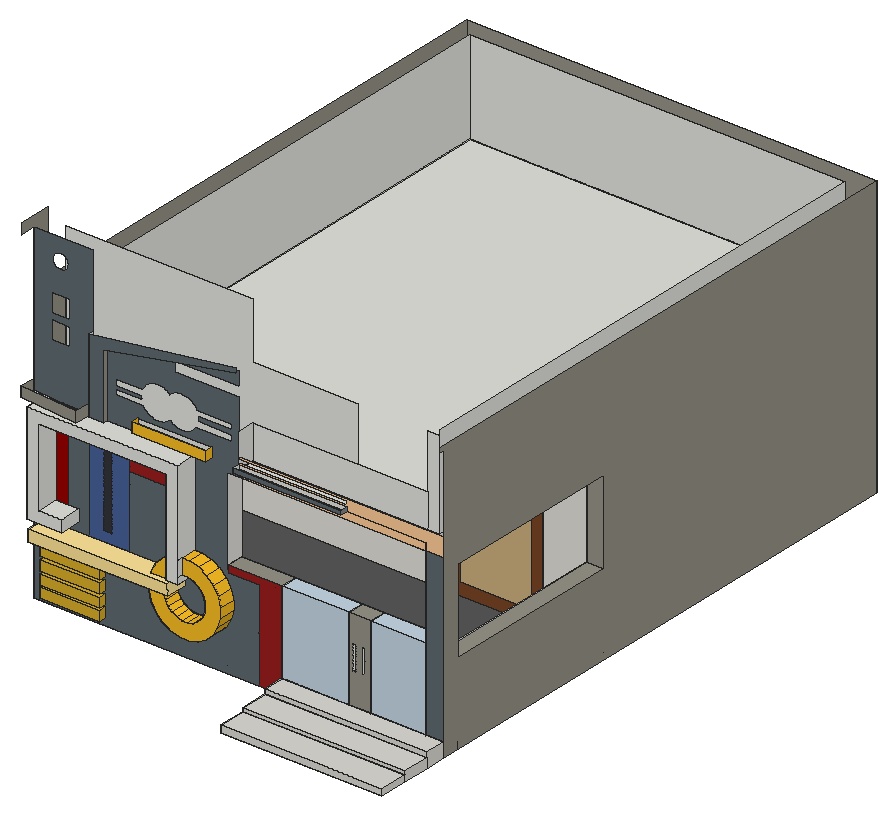
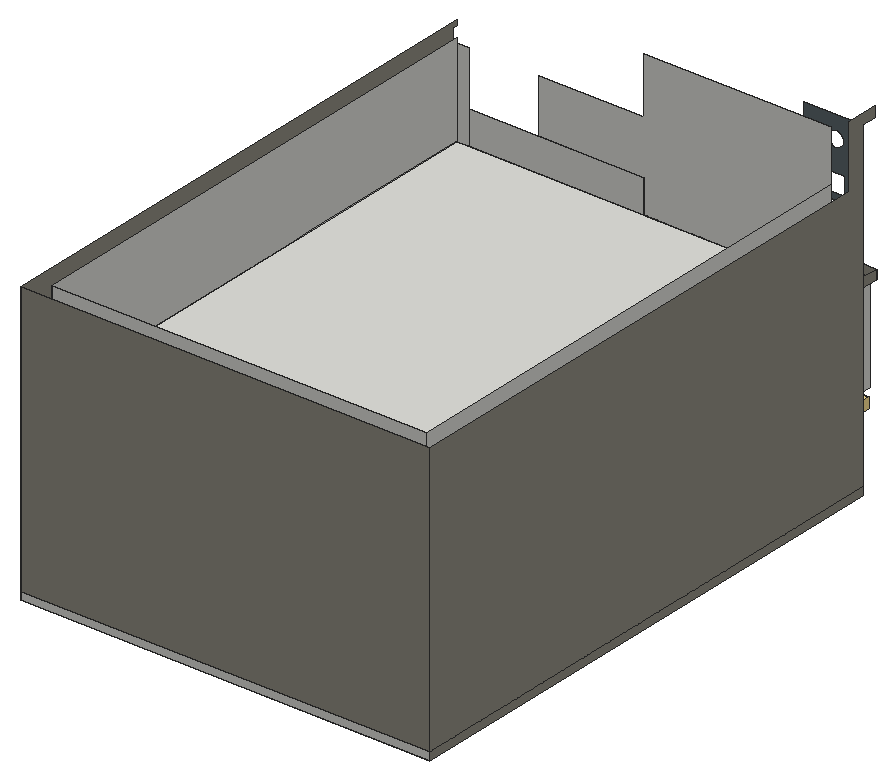
# SketchUp Ruby script. Lengths in inches.
U = 1.inch
M = Sketchup.active_model
def pt(a) = Geom::Point3d.new(a.map { |v| v * U })
def face(e, loops, mat)
  f = e.add_face(loops[0].map { |a| pt(a) })
  loops[1..].each { |l| e.add_face(l.map { |a| pt(a) }).erase! }
  f.material = f.back_material = mat if mat
  f
end
# faces: each face lists its corners as indices into pts; further lists are holes
def faces(e, pts, list, mat = nil) = list.each { |f| face(e, (f[0].is_a?(Array) ? f : [f]).map { |l| l.map { |i| pts[i] } }, mat) }
# xy, xz, yz: faces in a plane at the given z, y or x. An outline is a flat list of corners, or four numbers for a rectangle; further outlines are holes
def ring(l) = l.size == 4 ? [[l[0], l[1]], [l[2], l[1]], [l[2], l[3]], [l[0], l[3]]] : l.each_slice(2).to_a
def flat(e, list, mat, &to3) = list.each { |f| face(e, (f[0].is_a?(Array) ? f : [f]).map { |l| ring(l).map { |u, v| to3.(u, v) } }, mat) }
def xy(e, z, list, mat = nil) = flat(e, list, mat) { |x, y| [x, y, z] }
def xz(e, y, list, mat = nil) = flat(e, list, mat) { |x, z| [x, y, z] }
def yz(e, x, list, mat = nil) = flat(e, list, mat) { |y, z| [x, y, z] }
def lines(e, pts, list) = list.each { |a, b| e.add_line(pt(pts[a]), pt(pts[b])) }
# prism: a flat outline (further loops are holes) pulled along v
def prism(e, loops, v, mat = nil)
  f = face(e, loops, mat); d = Geom::Vector3d.new(v.map { |x| x * U })
  f.pushpull(f.normal.samedirection?(d) ? d.length : -d.length)
end
def box(e, o, s, mat = nil) = prism(e, [[o, [o[0] + s[0], o[1], o[2]], [o[0] + s[0], o[1] + s[1], o[2]], [o[0], o[1] + s[1], o[2]]]], [0, 0, s[2]], mat)
def at(x, y, z, deg = 0) = Geom::Transformation.translation(pt([x, y, z])) * Geom::Transformation.rotation(ORIGIN, Z_AXIS, deg.degrees)
def axes(o, x, y, z) = Geom::Transformation.new([*x, 0, *y, 0, *z, 0, *pt(o).to_a, 1])
def part(name) = M.definitions.add(name)
# library, detail: a bought-in or finely detailed component or shape, given as its bounding box
def library(name, o, s) = part(name).tap { |d| box(d.entities, o, s) }
def detail(e, o, s) = box(e.add_group.entities, o, s)
def put(e, d, t, mat = nil) = e.add_instance(d, t).tap { |i| i.material = mat if mat }
def group(e, t, mat = nil) = e.add_group.tap { |g| g.transformation = t; g.material = mat if mat }.entities
root = M.entities
M.materials.add("[0045_Goldenrod]").color = [249, 189, 36]
M.materials.add("[Blacktop Old 01]").color = [132, 136, 139]
M.materials.add("[Carpet Plush Charcoal]").color = [87, 87, 87]
M.materials.add("[Color A04]").color = [155, 30, 30]
M.materials.add("[Color A07]").color = [153, 0, 0]
M.materials.add("[Color C02]").color = [255, 204, 153]
M.materials.add("[Color D02]").color = [255, 229, 153]
M.materials.add("[Color D04]").color = [216, 173, 42]
M.materials.add("[Formica Blue]").color = [71, 97, 152]
M.materials.add("[Formica Graystone]").color = [149, 146, 135]
M.materials.add("[Formica Laminate Dark]").color = [50, 53, 60]
M.materials.add("[Formica Speckled Grey]").color = [94, 105, 111]
M.materials.add("[Marble Carrara Gold Floor Tile]").color = [225, 223, 217]
M.materials.add("[Terrazzo Light Blue]").color = [196, 214, 227]
M.materials.add("[Terrazzo Tile Light]").color = [219, 217, 210]
M.materials.add("[Window Covering 02]").color = [199, 178, 115]
M.materials.add("[Wood Bamboo]").color = [177, 105, 43]
M.materials.add("[Wood Floor Light]").color = [204, 176, 127]
M.materials.add("[Wood Veneer 01]").color = [120, 70, 37]
M.materials.add("[Wood Veneer 02]").color = [190, 128, 91]
xy(root,0,[[307.14,0,506.36,34.29],[307.14,34.29,506.36,68.57],[307.14,68.57,506.36,94.74],[1.43,94.74,506.36,761.28]])
xy(root,7.65,[[14.67,86.37,88.61,94.74]])
xy(root,8.0625,[[307.14,0,506.36,34.29]],"[Terrazzo Tile Light]")
xy(root,9,[[307.14,94.74,389.07,116.19],[389.07,94.74,416.47,116.19],[416.47,94.74,484.91,116.19],[22.875,341.3,314.74,362.64],[314.74,341.3,431.36,362.64],
  [431.36,341.3,484.91,362.64],[22.875,362.64,484.91,739.83]])
xy(root,9,[[22.875,116.19,484.91,341.3]],"[Carpet Plush Charcoal]")
xy(root,12.25,[[307.14,34.29,506.36,68.57]],"[Terrazzo Tile Light]")
xy(root,18.125,[[307.14,68.57,506.36,94.74]],"[Terrazzo Tile Light]")
xy(root,19.77,[[14.67,86.37,88.61,94.74]],"[Color D04]")
xy(root,22.33,[[14.67,86.37,88.61,94.74]])
xy(root,34.46,[[14.67,86.37,88.61,94.74]],"[Color D04]")
xy(root,38.08,[[14.67,86.37,88.61,94.74]])
xy(root,50.21,[[14.67,86.37,88.61,94.74]],"[Color D04]")
xy(root,53.83,[[14.67,86.37,88.61,94.74]])
xy(root,65.96,[[14.67,86.37,88.61,94.74]],"[Color D04]")
xy(root,78.48,[[15.3,67.74,158.3125,94.74],[158.3125,67.74,177.44,75.3],[177.44,67.74,187.4,94.74]])
xy(root,89.58,[[129.59,341.3,239.96,362.64]])
xy(root,92.04,[[15.3,67.74,187.09,67.74,187.09,94.74,181.82,94.74,181.82,75.3,160.61,75.3,160.61,94.74,15.3,94.74]],"[Color D02]")
xy(root,96,[[185.25,67.74,199.68,94.74]])
xy(root,101,[[484.91,116.19,506.36,341.3]],"[Formica Graystone]")
xy(root,103.04,[[14.18,67.74,56.82,94.74]])
xy(root,117.47,[[28.61,67.74,56.82,94.74]])
xy(root,119.8125,[[240.02,94.74,307.14,116.19],[389.07,94.74,416.47,116.19]],"[Formica Graystone]")
xy(root,119.8125,[[307.14,94.74,389.07,116.19],[416.47,94.74,484.91,116.19]],"[Terrazzo Light Blue]")
xy(root,191.83,[[129.59,341.3,239.96,362.64]])
xy(root,197.7,[[314.74,341.3,431.36,362.64]])
xy(root,205.0625,[[484.91,116.19,506.36,341.3]],"[Formica Graystone]")
xy(root,212.8,[[28.61,67.74,44.09,94.74],[44.09,67.74,69.22,94.74],[69.22,67.74,118.93,94.74],[118.93,67.74,185.25,94.74]])
xy(root,221.375,[[253.89,94.74,253.89,116.19,22.875,116.19,22.875,341.3,484.91,341.3,484.91,94.74],[240.02,94.74,253.89,116.19],[22.875,341.3,484.91,362.64],[22.875,362.64,484.91,739.83]])
xy(root,227.23,[[14.18,67.74,199.68,67.74,199.68,94.74,91.53,94.74,91.53,89.43,73.65,89.43,14.18,93.8],[73.65,89.43,73.65,94.74,14.18,94.74,14.18,93.8],[73.65,89.43,91.53,94.74]])
xy(root,230.375,[[253.89,94.74,470.23,116.19],[470.23,94.74,484.91,116.19],[22.875,116.19,484.91,739.83]])
xy(root,230.375,[[253.89,85.74,386.77,94.74]],"[Blacktop Old 01]")
xy(root,230.54,[[129.08,85.18,220.21,94.74]],"[0045_Goldenrod]")
xz(root,0,[[307.14,0,506.36,8.0625]],"[Terrazzo Tile Light]")
xz(root,34.29,[[307.14,0,506.36,8.0625]])
xz(root,34.29,[[307.14,8.0625,506.36,12.25]],"[Terrazzo Tile Light]")
xz(root,67.74,[[185.25,96,199.68,96,199.68,227.23,14.18,227.23,14.18,103.04,56.82,103.04,56.82,117.47,28.61,117.47,28.61,212.8,185.25,212.8]])
xz(root,67.74,[[15.3,78.48,187.4,78.48,187.09,92.04,15.3,92.04]],"[Color D02]")
xz(root,68.57,[[307.14,0,506.36,12.25]])
xz(root,68.57,[[307.14,12.25,506.36,18.125]],"[Terrazzo Tile Light]")
xz(root,75.3,[[208.09,33.22,219.43,36.12,229.62,41.86,237.98,50.04,243.94,60.1,247.1,71.37,247.22,83.07,244.32,94.4,238.58,104.6,230.4,112.96,220.34,118.92,209.07,122.07,199.68,122.17,199.68,103.04,206.34,102.97,212.76,101.17,218.49,97.78,223.15,93.02,226.41,87.21,228.07,80.76,227.99,74.1,226.2,67.68,222.81,61.95,218.04,57.29,212.24,54.03,205.79,52.375,199.125,52.45,192.71,54.24,186.98,57.64,182.32,62.4,179.05,68.2,177.4,74.66,177.44,78.48,158.3125,78.48,158.24,72.35,161.15,61.02,166.88,50.82,175.0625,42.46,185.13,36.5,196.4,33.35],[160.61,92.04,181.82,92.04,182.66,93.46,185.25,96,185.25,118.85,175.85,113.56,167.48,105.38,166.1,103.04,161.52,95.3125]],"[0045_Goldenrod]")
xz(root,85.18,[[129.08,230.54,220.21,243.23]],"[0045_Goldenrod]")
xz(root,85.74,[[253.89,230.375,386.77,235.375]],"[Formica Speckled Grey]")
xz(root,86.37,[[14.67,7.65,88.61,19.77],[14.67,22.33,88.61,34.46],[14.67,38.08,88.61,50.21],[14.67,53.83,88.61,65.96]],"[Color D04]")
xz(root,89.43,[[73.65,227.23,91.53,227.23,91.53,307.22,253.89,338.91,253.89,345.125,73.65,318.75]],"[Formica Speckled Grey]")
xz(root,94.74,[[[208.09,33.22,219.43,36.12,229.62,41.86,237.98,50.04,243.94,60.1,247.1,71.37,247.22,83.07,244.32,94.4,238.58,104.6,230.4,112.96,220.34,118.92,209.07,122.07,199.68,122.17,199.68,227.23,14.18,227.23,14.18,103.04,56.82,103.04,56.82,117.47,28.61,117.47,28.61,212.8,185.25,212.8,185.25,118.85,175.85,113.56,167.48,105.38,166.1,103.04,161.52,95.3125,160.61,92.04,15.3,92.04,15.3,78.48,158.3125,78.48,158.24,72.35,161.15,61.02,166.88,50.82,175.0625,42.46,185.13,36.5,196.4,33.35],[205.79,52.375,199.125,52.45,192.71,54.24,186.98,57.64,182.32,62.4,179.05,68.2,177.4,74.66,177.44,78.48,187.4,78.48,187.09,92.04,181.82,92.04,182.66,93.46,185.25,96,199.68,96,199.68,103.04,206.34,102.97,212.76,101.17,218.49,97.78,223.15,93.02,226.41,87.21,228.07,80.76,227.99,74.1,226.2,67.68,222.81,61.95,218.04,57.29,212.24,54.03]],[394.31,57.13,398.19,87.45],[405.38,57.13,409.25,87.45],[253.89,230.375,386.77,235.375]])
xz(root,94.74,[[278.8125,0,307.14,0,307.14,119.8125,240.02,119.8125,240.02,111.5,278.8125,111.5],[118.93,179.99,185.25,212.8]],"[Color A04]")
xz(root,94.74,[[28.61,117.47,44.09,212.8]],"[Color A07]")
xz(root,94.74,[[253.89,221.375,484.91,230.375],[484.91,221.375,506.36,221.375,506.36,243.88,253.89,243.88,253.89,242.13,386.77,242.13,386.77,237.13,253.89,237.13,253.89,235.375,386.77,235.375,386.77,230.375,484.91,230.375]],"[Color C02]")
xz(root,94.74,[[[69.22,92.04,118.93,212.8],[86.91,104.33,97.34,197.21]]],"[Formica Blue]")
xz(root,94.74,[[389.07,9,416.47,18.125],[[389.07,18.125,416.47,119.8125],[394.31,57.13,398.19,87.45],[405.38,57.13,409.25,87.45]]],"[Formica Graystone]")
xz(root,94.74,[[86.91,104.33,97.34,197.21]],"[Formica Laminate Dark]")
xz(root,94.74,[[[1.43,0,278.8125,0,278.8125,111.5,240.02,111.5,240.02,221.375,253.89,221.375,253.89,310.29,175.33,310.29,175.33,322.92,253.89,322.92,253.89,338.91,91.53,307.22,91.53,227.23,199.68,227.23,199.68,122.17,209.07,122.07,220.34,118.92,230.4,112.96,238.58,104.6,244.32,94.4,247.22,83.07,247.1,71.37,243.94,60.1,237.98,50.04,229.62,41.86,219.43,36.12,208.09,33.22,196.4,33.35,185.13,36.5,175.0625,42.46,166.88,50.82,161.15,61.02,158.24,72.35,158.3125,78.48,15.3,78.48,15.3,92.04,69.22,92.04,69.22,212.8,44.09,212.8,44.09,117.47,56.82,117.47,56.82,103.04,14.18,103.04,14.18,227.23,73.65,227.23,73.65,408.81,1.43,408.81],[153.66,248.1,151.5,248.25,149.38,248.64,147.3,249.24,145.31,250.05,143.4,251.07,141.62,252.28,139.97,253.68,138.47,255.23,137.15,256.9375,136.0625,258.6875,102.1,258.6875,102.1,265.74,133.7,265.74,133.53,266.98,133.46,269.14,133.48,269.39,101.95,269.39,101.95,276.95,135.19,276.95,135.41,277.49,136.43,279.39,137.64,281.18,139.04,282.83,140.59,284.32,142.3,285.65,144.13,286.79,146.08,287.73,148.11,288.46,150.2,288.98,152.34,289.27,154.5,289.34,156.65,289.18,158.78,288.8,160.85,288.2,162.85,287.38,164.75,286.36,166.54,285.15,168.19,283.76,168.82,283.1,170.09,284.32,171.8,285.65,173.63,286.79,175.58,287.73,177.61,288.46,179.7,288.98,181.84,289.27,184,289.34,186.15,289.18,188.28,288.8,190.35,288.2,192.35,287.38,194.25,286.36,196.04,285.15,197.69,283.76,199.19,282.2,200.51,280.5,201.65,278.66,202,277.9375,245.58,277.9375,245.58,270.5625,204.12,270.5625,204.13,270.45,204.2,268.3,204.08,266.6,204.04,266.14,203.97,265.74,245.58,265.74,245.58,257.2,200.65,257.2,200.01,256.26,198.62,254.61,197.0625,253.11,195.36,251.79,193.52,250.65,191.58,249.71,189.55,248.98,187.45,248.46,185.3125,248.17,183.16,248.1,181,248.25,178.88,248.64,176.8,249.24,174.81,250.05,172.9,251.07,171.12,252.28,169.47,253.68,168.84,254.33,167.5625,253.11,165.86,251.79,164.02,250.65,162.08,249.71,160.05,248.98,157.95,248.46,155.8125,248.17],[129.08,230.54,220.21,243.23],[14.67,53.83,88.61,65.96],[14.67,38.08,88.61,50.21],[14.67,22.33,88.61,34.46],[14.67,7.65,88.61,19.77],[23.1,292.05,45.78,314.74],[23.1,322.3,45.78,344.99],[34.11,372.72,31.62,373.05,29.3,374.01,27.3,375.54,25.78,377.53,24.8125,379.85,24.49,382.34,24.8125,384.83,25.78,387.15,27.3,389.15,29.3,390.68,31.62,391.64,34.11,391.97,36.6,391.64,38.92,390.68,40.92,389.15,42.45,387.15,43.41,384.83,43.74,382.34,43.41,379.85,42.45,377.53,40.92,375.54,38.92,374.01,36.6,373.05]],[307.14,0,506.36,9],[484.91,9,506.36,18.125],[484.91,18.125,506.36,221.375],[205.79,52.375,212.24,54.03,218.04,57.29,222.81,61.95,226.2,67.68,227.99,74.1,228.07,80.76,226.41,87.21,223.15,93.02,218.49,97.78,212.76,101.17,206.34,102.97,199.68,103.04,199.68,96,185.25,96,182.66,93.46,181.82,92.04,187.09,92.04,187.4,78.48,177.44,78.48,177.4,74.66,179.05,68.2,182.32,62.4,186.98,57.64,192.71,54.24,199.125,52.45],
  [118.93,92.04,160.61,92.04,161.52,95.3125,166.1,103.04,167.48,105.38,175.85,113.56,185.25,118.85,185.25,179.99,118.93,179.99]],"[Formica Speckled Grey]")
xz(root,94.74,[[307.14,9,389.07,18.125],[416.47,9,484.91,18.125],[307.14,18.125,389.07,119.8125],[416.47,18.125,484.91,119.8125]],"[Terrazzo Light Blue]")
xz(root,116.19,[[484.91,9,506.36,101],[22.875,221.375,253.89,230.375],[22.875,230.375,22.875,408.81,253.89,408.81,253.89,338.91,383.64,338.91,383.64,271.875,253.89,271.875,253.89,230.375],[253.89,230.375,470.23,271.875],[470.23,230.375,484.91,338.91]])
xz(root,116.19,[[389.07,9,416.47,119.8125],[484.91,101,506.36,205.0625]],"[Formica Graystone]")
xz(root,116.19,[[307.14,9,389.07,119.8125],[416.47,9,484.91,119.8125]],"[Terrazzo Light Blue]")
xz(root,116.19,[[22.875,9,240.02,221.375],[240.02,9,240.02,115.1875,298.8125,115.1875,298.8125,119.8125,307.14,119.8125,307.14,9],[240.02,115.1875,298.8125,119.8125]],"[Wood Bamboo]")
xz(root,341.3,[[336.71,84.47,341.96,119.4],[484.91,101,506.36,205.0625]],"[Formica Graystone]")
xz(root,341.3,[[[22.875,9,314.74,9,314.74,197.7,431.36,197.7,431.36,9,484.91,9,484.91,221.375,22.875,221.375],[129.59,89.58,239.96,191.83]]],"[Marble Carrara Gold Floor Tile]")
xz(root,341.3,[[138.99,98.98,177.99,182.43],[187.0625,98.98,230.5625,182.43]],"[Window Covering 02]")
xz(root,341.3,[[[329.99,24.26,416.1,182.45],[336.71,84.47,341.96,119.4]]],"[Wood Floor Light]")
xz(root,341.3,[[[314.74,9,431.36,197.7],[329.99,24.26,416.1,182.45]]],"[Wood Veneer 01]")
xz(root,341.3,[[[129.59,89.58,239.96,191.83],[138.99,98.98,230.5625,182.43]],[177.99,98.98,187.0625,182.43]],"[Wood Veneer 02]")
xz(root,362.64,[[[22.875,9,22.875,221.375,484.91,221.375,484.91,9,431.36,9,431.36,197.7,314.74,197.7,314.74,9],[129.59,89.58,239.96,191.83]]])
xz(root,739.83,[[22.875,9,484.91,221.375],[22.875,221.375,484.91,230.375],[22.875,230.375,484.91,345.125]])
xz(root,761.28,[[1.43,0,506.36,9]])
xz(root,761.28,[[1.43,9,506.36,345.125]],"[Formica Graystone]")
yz(root,1.43,[[94.74,0,761.28,9],[94.74,9,94.74,408.81,76.18,408.81,76.18,421.875,116.19,421.875,116.19,345.125,761.28,345.125,761.28,9]],"[Formica Graystone]")
yz(root,14.18,[[67.74,103.04,94.74,227.23]])
yz(root,14.67,[[86.37,7.65,94.74,19.77],[86.37,22.33,94.74,34.46],[86.37,38.08,94.74,50.21],[86.37,53.83,94.74,65.96]],"[Color D04]")
yz(root,15.3,[[67.74,78.48,94.74,92.04]],"[Color D02]")
yz(root,22.875,[[341.3,9,362.64,221.375],[362.64,9,739.83,221.375],[116.19,221.375,341.3,230.375],[341.3,221.375,362.64,230.375],[362.64,221.375,739.83,230.375],
  [116.19,230.375,739.83,345.125]])
yz(root,22.875,[[116.19,9,341.3,221.375]],"[Wood Bamboo]")
yz(root,28.61,[[67.74,117.47,94.74,212.8]])
yz(root,56.82,[[67.74,103.04,94.74,117.47]])
yz(root,73.65,[[89.43,227.23,94.74,318.75]])
yz(root,88.61,[[86.37,7.65,94.74,19.77],[86.37,22.33,94.74,34.46],[86.37,38.08,94.74,50.21],[86.37,53.83,94.74,65.96]],"[Color D04]")
yz(root,91.53,[[89.43,227.23,94.74,307.22]],"[Formica Graystone]")
yz(root,129.08,[[85.18,230.54,94.74,243.23]],"[0045_Goldenrod]")
yz(root,129.59,[[341.3,89.58,362.64,191.83]])
yz(root,185.25,[[67.74,96,75.3,118.85],[67.74,118.85,94.74,179.99],[67.74,179.99,94.74,212.8]])
yz(root,199.68,[[67.74,96,94.74,103.04],[67.74,103.04,75.3,122.17],[67.74,122.17,94.74,227.23]])
yz(root,220.21,[[85.18,230.54,94.74,243.23]],"[0045_Goldenrod]")
yz(root,239.96,[[341.3,89.58,362.64,191.83]])
yz(root,240.02,[[94.74,115.1875,116.19,119.8125]])
yz(root,240.02,[[94.74,119.8125,116.19,221.375]],"[Marble Carrara Gold Floor Tile]")
yz(root,253.89,[[94.74,221.375,116.19,230.375],[85.74,230.375,94.74,235.375],[94.74,230.375,116.19,271.875]])
yz(root,307.14,[[94.74,9,116.19,119.8125]])
yz(root,307.14,[[0,0,34.29,8.0625],[34.29,0,68.57,12.25],[68.57,0,94.74,18.125]],"[Terrazzo Tile Light]")
yz(root,314.74,[[341.3,9,362.64,197.7]])
yz(root,386.77,[[85.74,230.375,94.74,235.375]],"[Blacktop Old 01]")
yz(root,389.07,[[94.74,9,116.19,119.8125]])
yz(root,416.47,[[94.74,9,116.19,119.8125]])
yz(root,431.36,[[341.3,9,362.64,197.7]])
yz(root,484.91,[[94.74,9,116.19,119.8125],[116.19,9,341.3,101],[341.3,9,362.64,221.375],[362.64,9,739.83,221.375],[94.74,221.375,341.3,230.375],
  [341.3,221.375,362.64,230.375],[362.64,221.375,739.83,230.375],[116.19,230.375,739.83,345.125]])
yz(root,484.91,[[94.74,119.8125,94.74,221.375,341.3,221.375,341.3,205.0625,116.19,205.0625,116.19,119.8125]],"[Marble Carrara Gold Floor Tile]")
yz(root,506.36,[[[94.74,0,761.28,0,761.28,345.125,89.43,345.125,89.43,338.91,94.74,338.91],[116.19,101,341.3,205.0625]]],"[Formica Graystone]")
yz(root,506.36,[[0,0,34.29,8.0625],[34.29,0,68.57,12.25],[68.57,0,94.74,18.125]],"[Terrazzo Tile Light]")
p = [[196.4,94.74,33.35],[208.09,94.74,33.22],[208.09,75.3,33.22],[196.4,75.3,33.35],[219.43,94.74,36.12],[219.43,75.3,36.12],
  [185.13,94.74,36.5],[185.13,75.3,36.5],[229.62,94.74,41.86],[229.62,75.3,41.86],[175.0625,94.74,42.46],[175.0625,75.3,42.46],
  [237.98,94.74,50.04],[237.98,75.3,50.04],[166.88,94.74,50.82],[166.88,75.3,50.82],[243.94,94.74,60.1],[243.94,75.3,60.1],
  [161.15,94.74,61.02],[161.15,75.3,61.02],[199.125,94.74,52.45],[192.71,94.74,54.24],[192.71,75.3,54.24],[199.125,75.3,52.45],
  [205.79,94.74,52.375],[205.79,75.3,52.375],[212.24,94.74,54.03],[212.24,75.3,54.03],[218.04,94.74,57.29],[218.04,75.3,57.29],
  [186.98,94.74,57.64],[186.98,75.3,57.64],[222.81,94.74,61.95],[222.81,75.3,61.95],[182.32,94.74,62.4],[182.32,75.3,62.4],
  [247.1,94.74,71.37],[247.1,75.3,71.37],[158.24,94.74,72.35],[158.24,75.3,72.35],[226.2,94.74,67.68],[226.2,75.3,67.68],
  [179.05,94.74,68.2],[179.05,75.3,68.2],[227.99,94.74,74.1],[227.99,75.3,74.1],[177.4,94.74,74.66],[177.4,75.3,74.66],
  [247.22,94.74,83.07],[247.22,75.3,83.07],[158.3125,94.74,78.48],[158.3125,75.3,78.48],[228.07,94.74,80.76],[228.07,75.3,80.76],
  [177.44,94.74,78.48],[177.44,75.3,78.48],[187.4,94.74,78.48],[187.09,94.74,92.04],[187.09,67.74,92.04],[187.4,67.74,78.48],
  [226.41,94.74,87.21],[226.41,75.3,87.21],[244.32,94.74,94.4],[244.32,75.3,94.4],[223.15,94.74,93.02],[223.15,75.3,93.02],
  [161.52,94.74,95.3125],[160.61,94.74,92.04],[160.61,75.3,92.04],[161.52,75.3,95.3125],[181.82,94.74,92.04],[182.66,94.74,93.46],
  [182.66,75.3,93.46],[181.82,75.3,92.04],[218.49,94.74,97.78],[218.49,75.3,97.78],[185.25,94.74,96],[185.25,75.3,96],
  [238.58,94.74,104.6],[238.58,75.3,104.6],[166.1,94.74,103.04],[166.1,75.3,103.04],[212.76,94.74,101.17],[212.76,75.3,101.17],
  [206.34,94.74,102.97],[206.34,75.3,102.97],[167.48,94.74,105.38],[167.48,75.3,105.38],[199.68,94.74,103.04],[199.68,75.3,103.04],
  [230.4,94.74,112.96],[230.4,75.3,112.96],[175.85,94.74,113.56],[175.85,75.3,113.56],[220.34,94.74,118.92],[220.34,75.3,118.92],
  [185.25,94.74,118.85],[185.25,75.3,118.85],[209.07,94.74,122.07],[209.07,75.3,122.07],[199.68,94.74,122.17],[199.68,75.3,122.17],
  [73.65,89.43,227.23],[73.65,89.43,228.7],[1.43,94.74,229.74],[1.43,94.74,227.23],[14.18,93.8,227.23],[0,75.36,241.27],
  [0,75.36,229.74],[72.23,70.04,228.7],[72.23,70.04,241.27],[73.65,89.43,241.27],[1.43,94.74,241.27],[22.875,116.19,9],
  [22.875,94.74,9],[484.91,341.3,9],[506.36,341.3,9],[506.36,116.19,9],[506.36,116.19,0],[240.02,116.19,9],
  [240.02,94.74,9],[298.8125,116.19,115.1875],[298.8125,94.74,115.1875]]
faces(root,p,[[0,1,2,3],[1,4,5,2],[6,0,3,7],[4,8,9,5],[10,6,7,11],[8,12,13,9],[14,10,11,15],[12,16,17,13],
  [18,14,15,19],[20,21,22,23],[24,20,23,25],[26,24,25,27],[28,26,27,29],[21,30,31,22],[32,28,29,33],[30,34,35,31],
  [16,36,37,17],[38,18,19,39],[40,32,33,41],[34,42,43,35],[44,40,41,45],[42,46,47,43],[36,48,49,37],[50,38,39,51],
  [52,44,45,53],[46,54,55,47],[60,52,53,61],[48,62,63,49],[64,60,61,65],[66,67,68,69],[74,64,65,75],[62,78,79,63],
  [80,66,69,81],[82,74,75,83],[84,82,83,85],[86,80,81,87],[88,84,85,89],[78,90,91,79],[92,86,87,93],[90,94,95,91],
  [96,92,93,97],[94,98,99,95],[98,100,101,99]],"[0045_Goldenrod]")
faces(root,p,[[56,57,58,59]],"[Color D02]")
faces(root,p,[[70,71,72,73],[71,76,77,72],[102,103,104,105,106],[104,103,109,108]])
faces(root,p,[[107,108,109,110],[103,111,110,109],[112,104,108,107]],"[Formica Graystone]")
lines(root,p,[[113,114],[115,116],[117,118],[119,120],[121,122]])
